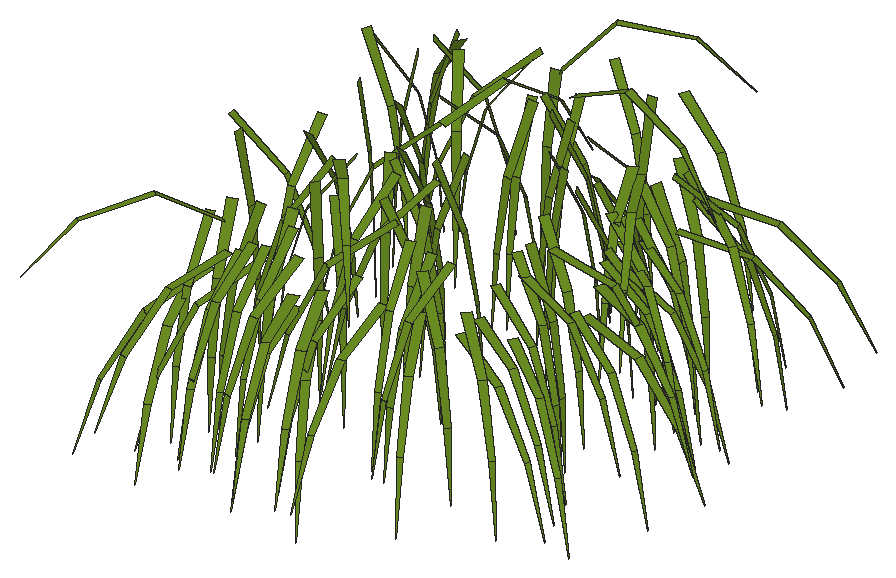
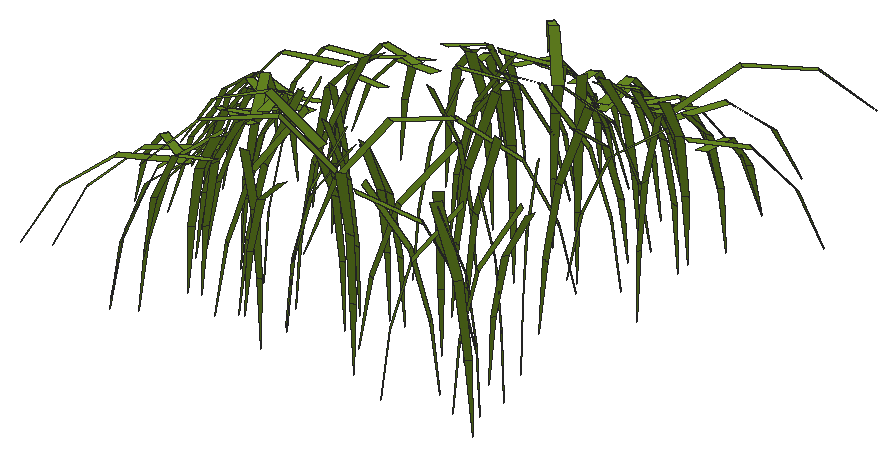
# SketchUp Ruby script. Lengths in inches.
U = 1.inch
M = Sketchup.active_model
def pt(a) = Geom::Point3d.new(a.map { |v| v * U })
def face(e, loops, mat)
  f = e.add_face(loops[0].map { |a| pt(a) })
  loops[1..].each { |l| e.add_face(l.map { |a| pt(a) }).erase! }
  f.material = f.back_material = mat if mat
  f
end
# faces: each face lists its corners as indices into pts; further lists are holes
def faces(e, pts, list, mat = nil) = list.each { |f| face(e, (f[0].is_a?(Array) ? f : [f]).map { |l| l.map { |i| pts[i] } }, mat) }
# xy, xz, yz: faces in a plane at the given z, y or x. An outline is a flat list of corners, or four numbers for a rectangle; further outlines are holes
def ring(l) = l.size == 4 ? [[l[0], l[1]], [l[2], l[1]], [l[2], l[3]], [l[0], l[3]]] : l.each_slice(2).to_a
def flat(e, list, mat, &to3) = list.each { |f| face(e, (f[0].is_a?(Array) ? f : [f]).map { |l| ring(l).map { |u, v| to3.(u, v) } }, mat) }
def xy(e, z, list, mat = nil) = flat(e, list, mat) { |x, y| [x, y, z] }
def xz(e, y, list, mat = nil) = flat(e, list, mat) { |x, z| [x, y, z] }
def yz(e, x, list, mat = nil) = flat(e, list, mat) { |y, z| [x, y, z] }
def lines(e, pts, list) = list.each { |a, b| e.add_line(pt(pts[a]), pt(pts[b])) }
# prism: a flat outline (further loops are holes) pulled along v
def prism(e, loops, v, mat = nil)
  f = face(e, loops, mat); d = Geom::Vector3d.new(v.map { |x| x * U })
  f.pushpull(f.normal.samedirection?(d) ? d.length : -d.length)
end
def box(e, o, s, mat = nil) = prism(e, [[o, [o[0] + s[0], o[1], o[2]], [o[0] + s[0], o[1] + s[1], o[2]], [o[0], o[1] + s[1], o[2]]]], [0, 0, s[2]], mat)
def at(x, y, z, deg = 0) = Geom::Transformation.translation(pt([x, y, z])) * Geom::Transformation.rotation(ORIGIN, Z_AXIS, deg.degrees)
def axes(o, x, y, z) = Geom::Transformation.new([*x, 0, *y, 0, *z, 0, *pt(o).to_a, 1])
def part(name) = M.definitions.add(name)
# library, detail: a bought-in or finely detailed component or shape, given as its bounding box
def library(name, o, s) = part(name).tap { |d| box(d.entities, o, s) }
def detail(e, o, s) = box(e.add_group.entities, o, s)
def put(e, d, t, mat = nil) = e.add_instance(d, t).tap { |i| i.material = mat if mat }
def group(e, t, mat = nil) = e.add_group.tap { |g| g.transformation = t; g.material = mat if mat }.entities
root = M.entities
M.materials.add("[0061_OliveDrab]").color = [107, 142, 35]
p = [[579.05,9.86,553.23],[578.98,9.68,553.23],[579.81,9.45,550.75],[571.21,2.62,553.25],[571.03,2.51,553.25],[571.64,1.73,550.82],
  [578.25,6.98,553.24],[578.15,6.81,553.24],[579.0625,6.37,550.82],[577.96,13.45,553.41],[577.95,13.24,553.41],[578.41,13.33,550.82],
  [577.97,18.34,553.38],[577.99,18.15,553.38],[578.41,18.29,550.79],[575.58,10.51,553.64],[575.52,10.32,553.64],[575.73,10.35,551.03],
  [576.31,16.2,553.59],[576.24,15.99,553.59],[576.47,16.04,550.97],[565.39,2.12,553.51],[565.19,2.05,553.51],[565.61,1.06,551.12],
  [563.21,2.34,553.51],[563.01,2.42,553.51],[562.75,1.44,551.09],[576.43,5.89,553.66],[576.3,5.72,553.66],[576.87,5.41,551.11],
  [565.49,5.79,553.6875],[565.28,5.8125,553.6875],[565.37,5.62,551.07],[577.625,14.6,553.66],[577.58,14.41,553.66],[578.01,14.41,551.07],
  [576.96,18.34,553.7],[576.98,18.12,553.7],[577.28,18.25,551.09],[564.86,4.23,553.8],[564.68,4.17,553.8],[564.9,3.78,551.21],
  [565.4,5.38,553.8],[565.2,5.3,553.8],[565.39,5.12,551.19],[576.98,13.33,553.81],[576.875,13.15,553.81],[577.24,13.05,551.21],
  [572.03,6.16,553.92],[571.83,6.14,553.92],[571.95,5.85,551.32],[574.2,6.41,553.86],[574.07,6.23,553.86],[574.46,6.09,551.26],
  [570.02,3.57,553.93],[569.83,3.57,553.93],[569.91,2.99,551.375],[567.27,5.6,554.02],[567.06,5.56,554.02],[567.22,5.32,551.41],
  [567.1875,8.64,554],[567.09,8.48,554],[567.17,8.54,551.375],[576.23,17.03,553.98],[576.12,16.85,553.98],[576.44,16.78,551.375],
  [574.36,3.79,553.99],[574.19,3.7,553.99],[574.72,2.95,551.53],[572.44,13.62,554.09],[572.26,13.66,554.09],[572.34,13.58,551.47],
  [574.67,14.91,554.09],[574.8,14.72,554.09],[574.86,14.9,551.47],[567.44,3.23,554.17],[567.26,3.18,554.17],[567.52,2.56,551.63],
  [567.47,4.39,554.14],[567.28,4.37,554.14],[567.42,3.93,551.56],[577.64,6.17,553.9375],[577.56,5.98,553.9375],[578.71,5.61,551.6],
  [568.94,7.67,554.19],[568.82,7.53,554.19],[568.98,7.51,551.57],[563.78,9.71,554.22],[563.77,9.5,554.22],[563.89,9.6,551.6],
  [579.99,10.95,553.94],[579.95,10.73,553.94],[581.21,10.61,551.64],[579.2,13.45,554.05],[579.18,13.26,554.05],[580.03,13.31,551.57],
  [575.63,14.9,554.24],[575.64,14.71,554.24],[575.86,14.82,551.62],[569.47,1.92,554.0625],[569.26,1.86,554.0625],[569.68,0.85,551.67],
  [565.27,2.67,554.22],[565.09,2.73,554.22],[564.92,1.93,551.73],[567.86,3.1,554.25],[567.63,3.1,554.25],[567.74,2.4,551.72],
  [571.13,8.18,554.3],[570.92,8.11,554.3],[571.09,7.9375,551.68],[576.43,9.14,554.29],[576.34,8.97,554.29],[576.79,8.85,551.7],
  [564.4375,14.73,554.28],[564.54,14.56,554.28],[564.53,14.67,551.65],[563.92,16.45,554.3125],[563.77,16.62,554.3125],[563.79,16.49,551.6875],
  [568.74,18.13,554.33],[568.52,18.1,554.33],[568.64,18.05,551.71],[572.16,18.64,554.27],[571.97,18.61,554.27],[572.08,18.53,551.65],
  [577.28,7.99,554.35],[577.21,7.82,554.35],[577.93,7.63,551.83],[568.37,10.46,554.4],[568.18,10.36,554.4],[568.32,10.32,551.78],
  [570.86,15.26,554.45],[570.67,15.3,554.45],[570.74,15.14,551.83],[566.18,15.27,554.44],[566.39,15.22,554.44],[566.32,15.37,551.82],
  [572.45,15.97,554.46],[572.62,15.86,554.46],[572.62,16.05,551.84],[573.72,17.05,554.36],[573.91,17.01,554.36],[573.88,17.36,551.76],
  [563.85,17.85,554.43],[563.71,17.97,554.43],[563.71,17.83,551.8],[577.28,18.94,554.34],[577.37,18.77,554.34],[577.76,19.07,551.76],
  [566.76,2.6,554.32],[566.55,2.54,554.32],[566.9,1.67,551.87],[571.36,9.27,554.54],[571.35,9.0625,554.54],[571.625,9.15,551.93],
  [575.9,10.97,554.54],[575.8,10.78,554.54],[576.2,10.6875,551.95],[569.35,11.25,554.55],[569.17,11.32,554.55],[569.2,11.12,551.93],
  [570.61,12.35,554.49],[570.66,12.16,554.49],[570.83,12.31,551.875],[568.16,13.34,554.54],[568.38,13.29,554.54],[568.31,13.5,551.93],
  [570.48,16.5,554.55],[570.28,16.48,554.55],[570.4,16.34,551.93],[570.75,2.46,554.31],[570.54,2.375,554.31],[571.09,1.33,551.97],
  [571.71,2.53,554.4],[571.5,2.5,554.4],[571.72,1.35,552.05],[565.17,12.54,554.64],[565.38,12.5,554.64],[565.32,12.77,552.03],
  [569.16,15.17,554.58],[568.93,15.19,554.58],[569.03,14.97,551.96],[569.6,15.31,554.66],[569.42,15.26,554.66],[569.57,15.0625,552.04],
  [571.53,17.57,554.58],[571.64,17.39,554.58],[571.77,17.59,551.97],[569.5,1.98,554.46],[569.28,1.91,554.46],[569.76,0.84,552.11],
  [566.5,2.73,554.5625],[566.48,2.72,554.5625],[566.72,1.87,552.09],[566.67,2.75,554.5625],[579.14,11.96,554.58],[579.09,11.78,554.58],
  [580.01,11.6,552.13],[563.93,18.55,554.74],[564.07,18.42,554.74],[564.15,18.65,552.125],[577.88,6.43,554.54],[577.79,6.25,554.54],
  [578.86,5.85,552.18],[579.12,13.36,554.66],[579.05,13.2,554.66],[580.02,12.87,552.24],[566.63,16.29,554.78],[566.47,16.17,554.78],
  [566.72,16,552.17],[564.13,16.7,554.77],[564.07,16.52,554.77],[564.38,16.52,552.16],[571.4,17.77,554.83],[571.43,17.57,554.83],
  [571.69,17.71,552.22],[565.05,9.4,554.88],[564.96,9.58,554.88],[564.73,9.36,552.28],[579.54,18.09,554.71],[579.61,17.9,554.71],
  [580.67,18.36,552.35],[565.4,18.15,554.88],[565.33,18.34,554.88],[565.08,18.16,552.27],[565.96,19.6,554.92],[566.1,19.42,554.92],
  [566.26,19.69,552.32],[572.22,5.31,554.94],[572.04,5.25,554.94],[572.34,4.73,552.39],[570.59,10.53,555.01],[570.54,10.36,555.01],
  [570.92,10.35,552.41],[562.72,19.47,554.96],[562.8125,19.67,554.96],[562.44,19.73,552.36],[572.78,4.91,555],[572.59,4.9,555],
  [572.73,4.22,552.47],[577.91,12.82,555.08],[577.83,12.64,555.08],[578.5,12.43,552.55],[573.33,18.62,555.0625],[573.52,18.51,555.0625],
  [573.625,18.92,552.47],[565.55,7.43,555.16],[565.375,7.51,555.16],[565.3,7.1,552.57],[564.58,1.87,555.06],[564.38,1.9,555.06],
  [564.3,0.65,552.75],[578.23,9.26,555.15],[578.19,9.0625,555.15],[579.08,8.94,552.68],[577.51,14.48,555.1875],[577.41,14.31,555.1875],
  [578.06,14.07,552.65],[568.14,17.73,555.28],[568.33,17.625,555.28],[568.45,18.04,552.69],[579.8,10.84,555.05],[579.72,10.64,555.05],
  [581.01,10.24,552.79],[578.99,15.9,555.2],[578.87,15.73,555.2],[579.89,15.17,552.85],[572.18,19.1,555.41],[572.08,18.94,555.41],
  [572.53,18.78,552.82],[565.1,9.01,555.43],[564.91,8.98,555.43],[565.09,8.53,552.85],[565.3,10.73,555.49],[565.32,10.55,555.49],
  [565.84,10.7,552.92],[568.3125,5.51,555.56],[568.12,5.63,555.56],[567.88,5,553.02],[565.4,11.6875,555.6],[565.28,11.83,555.6],
  [564.91,11.4,553.04],[568.85,7.16,555.67],[568.66,7.16,555.67],[568.76,6.61,553.1],[579.53,19.59,555.33],[579.59,19.39,555.33],
  [580.83,19.84,553.05],[576.83,7.89,555.25],[576.68,7.64,555.25],[577.65,10.48,555.36],[577.55,10.24,555.36],[565.375,16.83,555.74],
  [565.21,16.97,555.74],[564.95,16.46,553.18],[570.35,4.07,555.26],[570.1,3.92,555.26],[568.93,7.65,555.8125],[568.74,7.72,555.8125],
  [568.63,7.09,553.26],[578.9,11.79,555.59],[578.79,11.62,555.59],[579.92,11.01,553.3],[578.52,11.6,555.74],[578.52,11.375,555.74],
  [579.41,11.48,553.28],[576.97,13.53,555.84],[576.96,13.24,555.84],[577,18.26,555.82],[577.03,18.01,555.82],[564.91,3.81,555.46],
  [564.62,3.72,555.46],[563.86,3.87,555.54],[563.57,3.99,555.54],[576,19.2,556.08],[575.92,19.01,556.08],[576.6,18.84,553.55],
  [575.11,10.72,556.22],[575.02,10.44,556.22],[575.53,12.76,556.09],[575.35,12.67,556.09],[575.8,11.98,553.59],[575.8,16.4,556.16],
  [575.71,16.1,556.16],[575.4375,6.74,555.93],[575.25,6.5,555.93],[565.57,6.28,556.27],[565.28,6.31,556.27],[576.72,14.85,556.11],
  [576.66,14.59,556.11],[576.22,18.34,556.21],[576.24,18.03,556.21],[564.63,5.15,556.24],[564.38,5.08,556.24],[565.21,5.99,556.35],
  [564.93,5.875,556.35],[576.27,13.79,556.29],[576.12,13.54,556.29],[570.08,4.76,556.27],[569.82,4.76,556.27],[575.93,6.93,555.78],
  [575.82,6.66,555.78],[572.01,6.89,556.44],[571.72,6.86,556.44],[573.47,6.98,556.3125],[573.29,6.73,556.3125],[578.07,11.36,555.68],
  [578.01,11.05,555.68],[573.62,5.2,556.08],[573.38,5.07,556.08],[567.18,6.26,556.5625],[566.88,6.19,556.5625],[567.12,8.73,556.62],
  [566.98,8.49,556.62],[575.625,17.46,556.5],[575.46,17.2,556.5],[568.99,3.71,555.92],[568.69,3.62,555.92],[567.42,5.35,556.58],
  [567.15,5.33,556.58],[577.67,13.58,556.1875],[577.65,13.3125,556.1875],[572.53,13.79,556.71],[572.26,13.85,556.71],[574.28,14.7,556.67],
  [574.46,14.44,556.67],[565.79,4.11,556.36],[565.53,4.2,556.36],[567.14,4.53,556.43],[566.88,4.46,556.43],[568.68,7.96,556.79],
  [568.5,7.76,556.79],[563.53,9.76,556.84],[563.52,9.46,556.84],[575.03,14.91,556.79],[575.04,14.65,556.79],[570.1,4.15,556.22],
  [569.8125,4.03,556.22],[566.37,4.18,556.38],[566.08,4.1,556.38],[567.9,4.45,556.5],[567.58,4.45,556.5],[575.98,8.55,556.56],
  [575.88,8.3,556.56],[571.02,8.68,556.87],[570.72,8.59,556.87],[575.55,9.64,556.71],[575.43,9.4,556.71],[564.3,14.71,556.9],
  [564.44,14.45,556.9],[564.1,16.54,556.93],[563.88,16.78,556.93],[568.76,18.34,556.95],[568.45,18.3,556.95],[576.3125,18.52,556.74],
  [576.43,18.28,556.74],[572.17,18.89,556.89],[571.89,18.86,556.89],[571.57,4.33,556.3],[571.27,4.3,556.3],[568.27,10.74,557.01],
  [568.01,10.6,557.01],[566.06,14.95,557.05],[566.35,14.88,557.05],[573.53,16.35,556.88],[573.8,16.3,556.88],[564.09,18.0625,557.03],
  [563.9,18.23,557.03],[568.93,3.81,556.26],[568.63,3.71,556.26],[576.22,7.28,556.39],[576.1,7.03,556.39],[570.71,9.35,557.08],
  [570.69,9.05,557.08],[575.13,11.43,557.01],[574.99,11.16,557.01],[569.54,11.67,557.13],[569.27,11.76,557.13],[570.16,12.27,557.08],
  [570.24,11.99,557.08],[568,12.9,557.13],[568.32,12.82,557.13],[570.96,15.62,557.05],[570.7,15.67,557.05],[572.19,15.63,557.05],
  [572.4375,15.48,557.05],[566.45,4.3125,556.66],[566.19,4.27,556.66],[576.47,12.58,556.98],[576.3,12.47,556.98],[576.98,11.57,554.61],
  [577.56,12.48,556.61],[577.48,12.23,556.61],[565.02,11.98,557.2],[565.32,11.92,557.2],[569.25,15.67,557.15],[568.9375,15.7,557.15],
  [570.47,16.93,557.14],[570.19,16.9,557.14],[571.07,17.35,557.16],[571.23,17.08,557.16],[577.54,14.11,556.62],[577.43,13.875,556.62],
  [569.49,15.85,557.22],[569.23,15.77,557.22],[577.74,17.54,556.53],[577.83,17.26,556.53],[563.5,18.14,557.3],[563.71,17.95,557.3],
  [566.28,16.84,557.32],[566.05,16.67,557.32],[563.51,16.95,557.31],[563.42,16.68,557.31],[570.73,17.72,557.36],[570.77,17.4375,557.36],
  [571.82,6.46,557.27],[571.58,6.37,557.27],[565.71,9.67,557.41],[565.59,9.92,557.41],[566.08,18.33,557.41],[565.99,18.6,557.41],
  [565.38,19.21,557.45],[565.57,18.95,557.45],[572.73,6.29,557.23],[572.46,6.28,557.23],[569.82,10.78,557.51],[569.75,10.53,557.51],
  [577.9,11.66,556.66],[577.78,11.36,556.66],[563.4,19.08,557.46],[563.54,19.36,557.46],[564.92,3.82,556.79],[564.63,3.86,556.79],
  [576.64,9.7,557.18],[576.57,9.42,557.18],[576.67,13.44,557.3],[576.55,13.1875,557.3],[572.86,17.85,557.53],[573.12,17.71,557.53],
  [565.95,8.25,557.62],[565.7,8.36,557.62],[576.33,15.18,557.43],[576.2,14.93,557.43],[577.41,17.02,556.98],[577.25,16.78,556.98],
  [569.0625,6.21,556.08],[568.75,6.01,556.08],[574.73,9.19,556.14],[574.55,8.9,556.14],[567.63,16.95,557.73],[567.89,16.79,557.73],
  [577.57,19.11,557],[577.65,18.8125,557],[564.97,10.03,557.85],[564.7,9.98,557.85],[575.42,11.43,556.36],[575.29,11.13,556.36],
  [571.33,19.65,557.83],[571.19,19.43,557.83],[564.19,6.2,556.27],[563.84,6.09,556.27],[564.78,6.13,556.52],[564.43,6.27,556.52],
  [564.21,10.65,557.88],[564.24,10.39,557.88],[569.04,6.64,557.8125],[568.77,6.8,557.8125],[577.23,12.91,557.28],[577.08,12.68,557.28],
  [566.31,12.39,557.96],[566.13,12.6,557.96],[568.88,8.3125,558.02],[568.61,8.3125,558.02],[575.53,11.88,556.11],[575.46,11.5,556.11],
  [576.84,11.65,557.76],[576.83,11.34,557.76],[566.14,17.72,558.09],[565.9,17.91,558.09],[573.61,7.92,556.5],[573.48,7.59,556.5],
  [569.375,8.84,558.11],[569.11,8.93,558.11],[574.98,13.63,557.55],[574.97,13.27,557.55],[574.99,18.0625,557.49],[575.03,17.74,557.49],
  [568.29,6.21,556.3],[567.92,6.1,556.3],[573.62,8.22,557.11],[573.39,7.93,557.11],[572.46,7.33,557.08],[572.18,7.17,557.08],
  [574.875,14.2,558.18],[574.62,14.08,558.18],[574.8125,15.33,557.85],[574.74,15.01,557.85],[574.72,19.76,558.3],[574.61,19.5,558.3],
  [569.2,6.46,557.09],[568.84,6.3125,557.09],[564.1,7.04,557.99],[563.8,6.95,557.99],[573.82,11.2,558.45],[573.71,10.86,558.45],
  [575.24,13.75,557.16],[575.22,13.42,557.16],[574.43,16.85,558.35],[574.32,16.48,558.35],[574.52,18.26,558.21],[574.54,17.88,558.21],
  [568.14,6.28,556.64],[567.77,6.16,556.64],[571.35,6.8,557.16],[570.99,6.77,557.16],[570.16,6.97,557.68],[569.84,6.98,557.68],
  [565.72,7.57,558.55],[565.36,7.6,558.55],[571.9,8.14,558.06],[571.68,7.84,558.06],[574.67,14.77,558.13],[574.49,14.46,558.13],
  [565.76,6.57,557.29],[565.4,6.47,557.29],[566.59,6.45,557.25],[566.28,6.55,557.25],[566.57,6.79,557.63],[566.26,6.71,557.63],
  [564.66,7.48,558.4375],[564.32,7.35,558.4375],[564.49,6.95,557.87],[571.9,8.59,558.43],[571.55,8.56,558.43],[573.93,8.43,556.94],
  [573.77,8.12,556.94],[567.93,6.79,557.69],[567.53,6.79,557.69],[575.28,16.75,557],[575.39,16.41,557],[574.22,18.37,558.52],
  [574.02,18.05,558.52],[568.98,18.4375,558.83],[569.19,18.38,558.83],[569.4,19.66,556.55],[567.26,7.29,558.34],[566.92,7.26,558.34],
  [566.89,7.8,558.67],[566.52,7.72,558.67],[573.78,9.46,557.67],[573.66,9.16,557.67],[566.88,8.9,559.23],[566.71,8.62,559.23],
  [575.16,13.24,557.35],[575.0625,12.93,557.35],[575.23,15.17,557.26],[575.1,14.88,557.26],[566.09,6.74,557.59],[565.77,6.69,557.59],
  [573.74,10.61,558.34],[573.59,10.32,558.34],[575.48,12.67,556.84],[575.33,12.31,556.84],[573.25,14.0625,559],[573.47,13.74,559],
  [572.68,14.28,559.28],[572.36,14.36,559.28],[574.39,17.625,558.29],[574.53,17.33,558.29],[565.33,6.39,557.13],[564.99,6.4375,557.13],
  [567.86,8.72,559.16],[567.64,8.47,559.16],[562.97,9.81,559.4],[562.96,9.44,559.4],[573.51,14.87,558.93],[573.52,14.55,558.93],
  [561.84,2.91,558.65],[561.6875,3.02,558.65],[560.66,1.4,556.85],[570.7,9.84,559.2],[570.34,9.73,559.2],[563.98,14.56,559.5],
  [564.16,14.26,559.5],[573.19,14.88,559.03],[573.51,14.82,559.03],[564.51,16.87,559.5],[564.25,17.16,559.5],[568.71,18.94,559.5],
  [568.6875,18.94,559.5],[568.33,18.89,559.5],[572.11,19.57,559.42],[571.77,19.53,559.42],[570.05,6.45,559.06],[569.88,6.31,559.06],
  [571.03,5.17,557],[567.91,11.49,559.5],[567.59,11.32,559.5],[573.46,12.36,558.81],[573.29,12.03,558.81],[575.46,14.27,558.71],
  [575.22,14.12,558.71],[565.79,14.06,559.5],[566.16,13.97,559.5],[571.58,14.7,559.42],[571.88,14.51,559.42],[575.27,18.52,557.25],
  [575.07,18.22,557.25],[564.7,18.71,559.5],[564.47,18.92,559.5],[575.05,18.46,557.35],[575.15,18.1,557.35],[569.22,9.45,559.24],
  [569.2,9.08,559.24],[567.71,11.81,559.5],[568.09,11.72,559.5],[569.18,12.02,559.5],[569.28,11.68,559.5],[569.94,12.72,559.5],
  [569.61,12.84,559.5],[571.16,16.54,559.5],[570.83,16.6,559.5],[570.35,18.08,559.5],[570.05,18.04,559.5],[570.01,18.03,559.5],
  [572.61,8.69,558.28],[572.27,8.67,558.28],[574.18,10.35,557.83],[574.09,10.01,557.83],[564.75,10.75,559.5],[565.11,10.68,559.5],
  [569.4,16.84,559.5],[569.01,16.875,559.5],[569.18,17.11,559.5],[568.85,17.02,559.5],[570.04,16.76,559.5],[570.24,16.44,559.5],
  [571.04,8.57,558.63],[570.75,8.45,558.63],[575.05,14.35,557.5625],[574.87,14.0625,557.5625],[574.49,14.49,558.32],[574.34,14.18,558.32],
  [562.14,17.42,559.5],[562.04,17.09,559.5],[565.44,18.05,559.5],[565.16,17.84,559.5],[562.53,17.1,559.5],[562.77,16.875,559.5],
  [574.77,17.64,559.43],[574.75,17.43,559.43],[576.23,17.41,557.26],[567.15,10.34,559.5],[567,10.64,559.5],[574.25,16.36,558.49],
  [574.08,16.06,558.49],[569.22,17.54,559.5],[569.27,17.2,559.5],[567.6,18.78,559.5],[567.49,19.11,559.5],[568.17,11.24,559.5],
  [568.09,10.93,559.5],[571.92,16.26,559.39],[572.25,16.08,559.39],[564.0625,18.23,559.5],[564.3,17.92,559.5],[564.87,18.32,559.5],
  [565.04,18.67,559.5],[566.73,9.96,559.45],[566.66,9.99,559.45],[566.42,10.1,559.45],[566.61,15.29,559.5],[566.9375,15.1,559.5],
  [570.29,8.66,558.93],[569.96,8.85,558.93],[564.65,12.04,559.5],[564.33,11.99,559.5],[574.25,11.7,558.2],[574.25,11.3125,558.2],
  [569.61,20.73,559.5],[569.45,20.45,559.5],[564.68,6.8125,557.87],[564.41,7,557.87],[563.13,5.14,559.21],[563.35,4.99,559.21],
  [562.15,10.44,559.5],[562.19,10.13,559.5],[568.89,10.53,559.43],[568.5625,10.53,559.43],[567.96,13.72,559.5],[567.83,13.88,559.5],
  [567.75,13.98,559.5],[570.14,11,559.39],[569.82,11.11,559.39],[567.54,19.44,559.5],[567.24,19.67,559.5],[573.8,16.5,558.84],
  [573.49,16.35,558.84],[574.11,15.85,558.65],[572.49,20.7,559.32],[572.36,20.38,559.32],[574.1,16.51,558.64],[573.8,16.33,558.64],
  [568.39,16.33,560.28],[568.69,16.25,560.28],[568.52,8.27,560.18],[568.28,8.0625,560.18],[572.4375,21.25,561.05],[572.55,21.06,561.05],
  [574.125,22.11,559.23],[572.43,17.88,560.6],[572.4,17.57,560.6],[566.88,10.1875,559.45],[566.59,9.93,559.45],[567.74,13.91,559.5],
  [568.1,13.8125,559.5],[570.06,18.11,559.5],[570.03,17.73,559.5],[568.59,19.1,559.5],[568.79,18.77,559.5],[570.33,19.71,561.41],
  [570.17,19.98,561.41]]
faces(root,p,[[0,1,2],[3,4,5],[6,7,8],[9,10,11],[12,13,14],[15,16,17],[18,19,20],[21,22,23],
  [24,25,26],[27,28,29],[30,31,32],[33,34,35],[36,37,38],[39,40,41],[42,43,44],[45,46,47],
  [48,49,50],[51,52,53],[54,55,56],[57,58,59],[60,61,62],[63,64,65],[66,67,68],[69,70,71],
  [72,73,74],[75,76,77],[78,79,80],[81,82,83],[84,85,86],[87,88,89],[90,91,92],[93,94,95],
  [96,97,98],[99,100,101],[102,103,104],[105,106,107],[108,109,110],[111,112,113],[114,115,116],[117,118,119],
  [120,121,122],[123,124,125],[126,127,128],[129,130,131],[132,133,134],[135,136,137],[138,139,140],[141,142,143],
  [144,145,146],[147,148,149],[150,151,152],[153,154,155],[156,157,158],[159,160,161],[162,163,164],[165,166,167],
  [168,169,170],[171,172,173],[174,175,176],[177,178,179],[180,181,182],[183,184,185],[186,187,188],[189,190,191],
  [192,193,194,195],[196,197,198],[199,200,201],[202,203,204],[205,206,207],[208,209,210],[211,212,213],[214,215,216],
  [217,218,219],[220,221,222],[223,224,225],[226,227,228],[229,230,231],[232,233,234],[235,236,237],[238,239,240],
  [241,242,243],[244,245,246],[247,248,249],[250,251,252],[253,254,255],[256,257,258],[259,260,261],[262,263,264],
  [265,266,267],[268,269,270],[271,272,273],[274,275,276],[277,278,279],[280,281,282],[283,284,285],[286,287,288],
  [289,290,7,6],[291,292,1,0],[293,294,295],[296,297,4,3],[298,299,300],[301,302,303],[304,305,306],[307,308,10,9],
  [309,310,13,12],[311,312,22,21],[313,314,25,24],[315,316,317],[318,319,16,15],[320,321,322],[323,324,19,18],[325,326,28,27],
  [327,328,31,30],[329,330,34,33],[331,332,37,36],[333,334,40,39],[335,336,43,42],[337,338,46,45],[339,340,55,54],[341,342,82,81],
  [343,344,49,48],[345,346,52,51],[347,348,91,90],[349,350,67,66],[351,352,58,57],[353,354,61,60],[355,356,64,63],[357,358,100,99],
  [359,360,79,78],[361,362,94,93],[363,364,70,69],[365,366,73,72],[367,368,103,102],[369,370,76,75],[371,372,85,84],[373,374,88,87],
  [375,376,97,96],[377,378,172,171],[379,380,192,151,150],[381,382,106,105],[383,384,127,126],[385,386,109,108],[387,388,112,111],[389,390,115,114],
  [391,392,118,117],[393,394,121,120],[395,396,148,147],[397,398,124,123],[399,400,175,174],[401,402,130,129],[403,404,136,135],[405,406,142,141],
  [407,408,145,144],[409,410,190,189],[411,412,203,202],[413,414,154,153],[415,416,157,156],[417,418,160,159],[419,420,163,162],[421,422,166,165],
  [423,424,133,132],[425,426,139,138],[427,428,193,192,195],[429,430,431],[432,433,197,196],[434,435,178,177],[436,437,181,180],[438,439,169,168],
  [440,441,187,186],[442,443,206,205],[444,445,184,183],[446,447,221,220],[448,449,200,199],[450,451,209,208],[452,453,212,211],[454,455,215,214],
  [456,457,230,229],[458,459,218,217],[460,461,224,223],[462,463,227,226],[464,465,239,238],[466,467,233,232],[468,469,263,262],[470,471,236,235],
  [472,473,251,250],[474,475,254,253],[476,477,242,241],[478,479,245,244],[480,481,248,247],[482,483,257,256],[484,485,266,265],[486,487,297,296],
  [488,489,290,289],[490,491,260,259],[492,493,287,286],[494,495,272,271],[496,497,292,291],[498,499,269,268],[500,501,312,311],[502,503,314,313],
  [504,505,275,274],[506,507,278,277],[508,509,302,301],[510,511,281,280],[512,513,284,283],[514,515,348,347],[516,517,305,304],[518,519,294,293],
  [520,521,342,341],[522,523,299,298],[524,525,308,307],[526,527,310,309],[528,529,358,357],[530,531,326,325],[532,533,350,349],[534,535,321,320],
  [536,537,330,329],[538,539,316,315],[540,541,378,377],[542,543,334,333],[544,545,319,318],[546,547,362,361],[548,549,324,323],[550,551,332,331],
  [552,553,410,409],[554,555,400,399],[556,557,340,339],[558,559,328,327],[560,561,346,345],[562,563,338,337],[564,565,380,379],[566,567,368,367],
  [568,569,370,369],[570,571,572,336,335],[573,574,344,343],[575,576,412,411],[577,578,382,381],[579,580,447,446],[581,582,356,355],[583,584,585],
  [586,587,360,359],[588,589,352,351],[590,591,384,383],[592,593,354,353],[594,595,433,432],[596,597,443,442],[598,599,428,427],[600,601,388,387],
  [602,603,469,468],[604,605,366,365],[606,607,364,363],[608,609,396,395],[610,611,473,472],[612,613,372,371],[614,615,374,373],[616,617,376,375],
  [618,619,620],[621,622,386,385],[623,624,390,389],[625,626,406,405],[627,628,392,391],[629,630,631,394,393],[632,633,398,397],[634,635,636],
  [637,638,402,401],[639,640,416,415],[641,642,430,429],[643,644,404,403],[645,646,426,425],[647,648,485,484],[649,650,408,407],[651,652,493,492],
  [653,654,414,413],[655,656,422,421],[657,658,420,419],[659,660,418,417],[661,662,424,423],[663,664,665,439,438],[666,667,465,464],[668,669,475,474],
  [670,671,435,434],[672,673,437,436],[674,675,445,444],[676,677,441,440],[678,679,457,456],[680,681,509,508],[682,683,477,476],[684,685,453,452],
  [686,687,451,450],[688,689,449,448],[690,691,692],[693,694,459,458],[695,696,483,482],[697,698,455,454],[699,700,461,460],[701,702,467,466],
  [703,704,479,478],[705,706,463,462],[707,708,471,470],[709,710,711,481,480],[712,713,491,490],[714,715,507,506],[716,717,495,494],[718,719,517,516],
  [720,721,499,498],[722,572,723,724,725],[726,727,505,504],[728,729,513,512],[730,731,732,511,510],[733,734,523,522],[735,736,519,518],[737,738,535,534,739],
  [740,741,539,538],[725,724,619,618],[742,743,739,642,641],[744,745,584,583],[746,747,635,634],[748,749,750],[751,752,691,690],[753,710,754,747,746],
  [755,731,756,745,744],[757,664,758,752,751],[759,630,760,761,762],[762,761,749,748]],"[0061_OliveDrab]")
